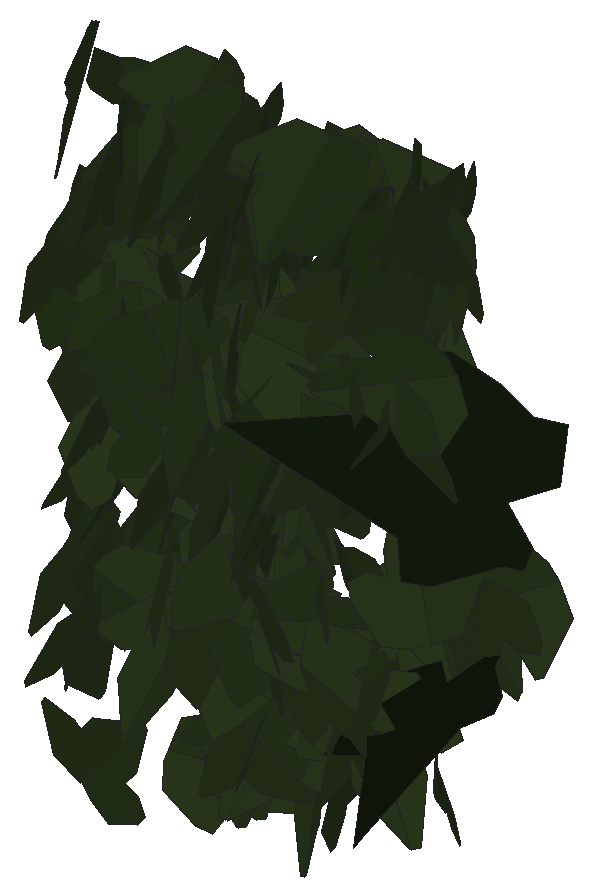
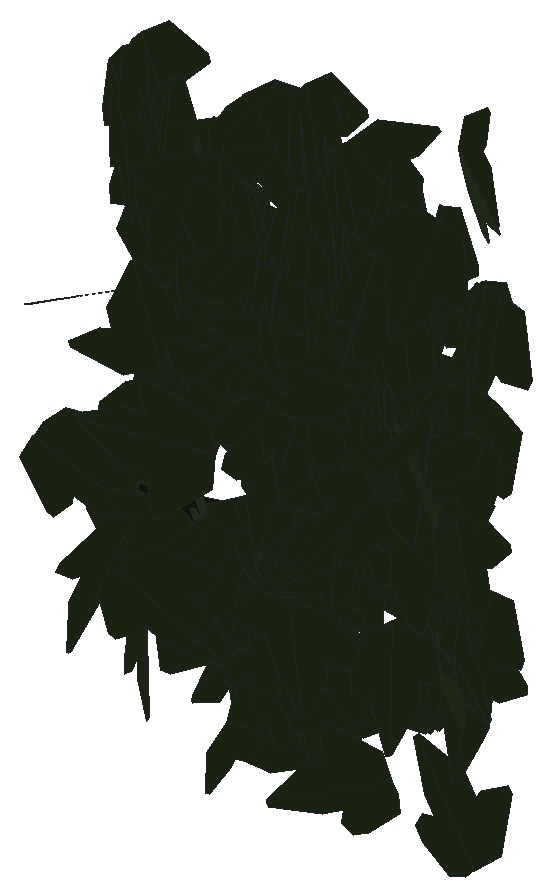
# SketchUp Ruby script. Lengths in inches.
U = 1.inch
M = Sketchup.active_model
def pt(a) = Geom::Point3d.new(a.map { |v| v * U })
def face(e, loops, mat)
  f = e.add_face(loops[0].map { |a| pt(a) })
  loops[1..].each { |l| e.add_face(l.map { |a| pt(a) }).erase! }
  f.material = f.back_material = mat if mat
  f
end
# faces: each face lists its corners as indices into pts; further lists are holes
def faces(e, pts, list, mat = nil) = list.each { |f| face(e, (f[0].is_a?(Array) ? f : [f]).map { |l| l.map { |i| pts[i] } }, mat) }
# xy, xz, yz: faces in a plane at the given z, y or x. An outline is a flat list of corners, or four numbers for a rectangle; further outlines are holes
def ring(l) = l.size == 4 ? [[l[0], l[1]], [l[2], l[1]], [l[2], l[3]], [l[0], l[3]]] : l.each_slice(2).to_a
def flat(e, list, mat, &to3) = list.each { |f| face(e, (f[0].is_a?(Array) ? f : [f]).map { |l| ring(l).map { |u, v| to3.(u, v) } }, mat) }
def xy(e, z, list, mat = nil) = flat(e, list, mat) { |x, y| [x, y, z] }
def xz(e, y, list, mat = nil) = flat(e, list, mat) { |x, z| [x, y, z] }
def yz(e, x, list, mat = nil) = flat(e, list, mat) { |y, z| [x, y, z] }
def lines(e, pts, list) = list.each { |a, b| e.add_line(pt(pts[a]), pt(pts[b])) }
# prism: a flat outline (further loops are holes) pulled along v
def prism(e, loops, v, mat = nil)
  f = face(e, loops, mat); d = Geom::Vector3d.new(v.map { |x| x * U })
  f.pushpull(f.normal.samedirection?(d) ? d.length : -d.length)
end
def box(e, o, s, mat = nil) = prism(e, [[o, [o[0] + s[0], o[1], o[2]], [o[0] + s[0], o[1] + s[1], o[2]], [o[0], o[1] + s[1], o[2]]]], [0, 0, s[2]], mat)
def at(x, y, z, deg = 0) = Geom::Transformation.translation(pt([x, y, z])) * Geom::Transformation.rotation(ORIGIN, Z_AXIS, deg.degrees)
def axes(o, x, y, z) = Geom::Transformation.new([*x, 0, *y, 0, *z, 0, *pt(o).to_a, 1])
def part(name) = M.definitions.add(name)
# library, detail: a bought-in or finely detailed component or shape, given as its bounding box
def library(name, o, s) = part(name).tap { |d| box(d.entities, o, s) }
def detail(e, o, s) = box(e.add_group.entities, o, s)
def put(e, d, t, mat = nil) = e.add_instance(d, t).tap { |i| i.material = mat if mat }
def group(e, t, mat = nil) = e.add_group.tap { |g| g.transformation = t; g.material = mat if mat }.entities
root = M.entities
M.materials.add("efeu1").color = [18, 25, 13]
M.materials.add("efeu2").color = [43, 57, 29]
c1 = part("ivyleaf_10")
p = [[0,0.5,-0.03],[-0.0625,2.02,-0.43],[-0.19,2.01,-0.46],[-0.54,1.05,-0.29],[-0.52,0.625,-0.18],[-0.83,0.76,-0.28],
  [-1.16,0.64,-0.33],[-1.15,0.33,-0.24],[-0.77,-0.39,0.02],[-0.3,-0.51,0.16],[0.04,-0.48,0.23],[-0.02,2.01,-0.4375],
  [-0.06,2.01,-0.43],[0.04,-0.49,0.23],[0.67,-0.49,0.14],[1.38,0.36,-0.2],[1.375,0.51,-0.24],[0.81,0.65,-0.19],
  [0.62,0.59,-0.15],[0.6,1.09,-0.28],[0.5,1.23,-0.31]]
faces(c1.entities,p,[[0,1,2,3,4,5,6,7,8,9,10],[11,12,0,13,14,15,16,17,18,19,20]],"efeu2")
c2 = part("ivyleaf_9")
p = [[1.54,2.16,1.25],[1.36,2.04,1.19],[-0.21,0.99,0.68],[-0.71,1.11,0.82],[-0.85,0.86,0.67],[-0.8,0.17,0.21],
  [-0.9,-0.01,0.1],[-0.67,-0.16,-0.02],[-0.08,-0.08,-0.05],[-0.03,-0.6,-0.4],[0.65,-0.88,-0.66],[0.83,-0.6,-0.49],
  [1.29,-0.42,-0.43],[1.8125,-0.07,-0.26],[1.21,0.44,0.15]]
faces(c2.entities,p,[[0,1,2,3,4,5,6,7,8,9,10,11,12,13,14]],"efeu1")
put(root,c1,axes([508.32,137.57,172.07],[0.33444,-0.46336,0.32616],[0.19775,-0.25949,-0.5714],[0.53102,0.38846,0.00736]))
put(root,c2,axes([512.88,137.89,165.84],[-0.5709,-0.44128,-0.42152],[0.64662,-0.3683,-0.39508],[0.02481,-0.55503,0.59729]))
put(root,c1,axes([513.1875,137.16,167.21],[0.1899,0.66022,-0.04458],[-0.01855,0.05168,0.68624],[0.66146,-0.18809,0.03204]))
put(root,c1,axes([511,137.58,168.73],[0.04279,-0.71118,0.27788],[0.07484,-0.27307,-0.7104],[0.75987,0.06694,0.05432]))
put(root,c2,axes([513.75,137.7,168.54],[-0.75068,0.35636,0.59387],[-0.70859,-0.54201,-0.47879],[0.16235,-0.71793,0.65625]))
put(root,c1,axes([510.41,136.8,166.26],[0.02054,-0.16896,-0.72847],[0.26646,0.68257,-0.15081],[0.69873,-0.25533,0.07892]))
put(root,c1,axes([511.78,137.48,169.28],[0.48375,-0.23299,0.34543],[0.34148,-0.08161,-0.53325],[0.23875,0.5888,0.06278]))
put(root,c1,axes([510.8,136.99,169.16],[-0.21497,0.24459,0.55114],[-0.42952,0.35297,-0.32478],[-0.46136,-0.44257,0.04557]))
put(root,c1,axes([511.97,137.625,165.58],[0.2065,-0.37848,-0.50768],[0.33346,-0.38896,0.42561],[-0.53832,-0.38612,0.06889]))
put(root,c1,axes([510.77,137.26,166.55],[-0.60109,0.4031,-0.03478],[0.02781,-0.02096,-0.72373],[-0.40364,-0.60173,0.00192]))
put(root,c1,axes([511.95,137.25,168.6],[-0.24629,-0.56282,-0.21689],[0.09421,0.19551,-0.61431],[0.59577,-0.26359,0.00747]))
put(root,c1,axes([509.11,137.61,167.84],[-0.25404,0.46707,0.36591],[0.11994,-0.3494,0.52927],[0.58109,0.27632,0.05073]))
put(root,c1,axes([510.3,137.42,170.68],[0.23232,-0.59093,-0.06122],[0.01744,0.07249,-0.63353],[0.59384,0.22905,0.04256]))
put(root,c1,axes([510.21,137.71,167.7],[0.13338,-0.60424,0.29815],[0.09615,-0.28376,-0.61808],[0.6669,0.16176,0.02948]))
put(root,c1,axes([511.46,137.47,165.78],[-0.28082,0.01322,-0.60596],[0.58482,-0.16953,-0.27472],[-0.15922,-0.646,0.05969]))
put(root,c1,axes([511,137.19,166.1875],[-0.31425,-0.21352,-0.5687],[0.51862,0.23908,-0.37634],[0.31629,-0.60416,0.05206]))
put(root,c1,axes([513.11,137.35,168.99],[-0.23811,0.01834,0.63],[-0.63026,-0.00386,-0.2381],[-0.00288,-0.67348,0.01852]))
put(root,c1,axes([512.95,137.49,169.77],[0.25306,0.09367,-0.64986],[-0.65654,0.04326,-0.24943],[0.00675,0.69605,0.10296]))
put(root,c1,axes([508.4,137.82,165.85],[0.24396,-0.4976,0.40781],[0.20164,-0.35503,-0.55383],[0.61095,0.31588,0.01995]))
put(root,c1,axes([510.9,137.26,164.86],[-0.34113,-0.40429,-0.35378],[0.24067,0.25966,-0.5288],[0.4803,-0.41725,0.01371]))
put(root,c1,axes([508.52,137.38,165.39],[-0.08968,-0.61593,-0.20414],[0.03086,0.2018,-0.62243],[0.64815,-0.09483,0.00139]))
put(root,c1,axes([509.37,137.84,165.36],[-0.23349,-0.48068,0.35286],[0.02561,-0.38668,-0.50981],[0.59574,-0.17177,0.16021]))
put(root,c1,axes([510.66,137.26,165.49],[0.27765,0.31305,0.44729],[0.24955,0.36454,-0.4196],[-0.51748,0.34376,0.03765]))
put(root,c1,axes([511.26,137.82,171.72],[-0.36212,-0.44252,0.31408],[-0.08731,-0.32515,-0.5588],[0.53558,-0.35221,0.12126]))
put(root,c1,axes([510.59,137.6,171.95],[0.06581,-0.66166,-0.0581],[0.00212,0.0586,-0.66488],[0.66421,0.06537,0.00788]))
put(root,c1,axes([508.23,137.41,170.1],[0.13259,-0.58806,-0.3005],[0.04504,0.31383,-0.59429],[0.65885,0.09689,0.1011]))
put(root,c1,axes([510.93,137.69,167.89],[0.3619,-0.12328,0.46846],[0.49098,-0.04076,-0.36333],[0.11542,0.55993,0.07669]))
put(root,c1,axes([512.94,137.65,171.84],[-0.00539,-0.64528,-0.01357],[0.00112,0.01356,-0.6453],[0.64542,-0.00541,0.00101]))
put(root,c1,axes([508.81,137.54,165.85],[-0.35451,-0.05588,-0.47064],[0.48814,0.03373,-0.34529],[0.065,-0.55803,0.02626]))
put(root,c1,axes([508.31,137.69,163.3],[-0.50719,-0.02251,0.41112],[0.40969,0.03734,0.50747],[-0.04098,0.65182,-0.01487]))
put(root,c1,axes([508.3,137.41,166.08],[-0.04211,-0.52875,-0.38857],[0.12038,0.37654,-0.52541],[0.64503,-0.10479,0.07269]))
put(root,c1,axes([511.05,137.87,171.66],[-0.26447,-0.53912,0.25266],[-0.05782,-0.2519,-0.59802],[0.59257,-0.26519,0.05441]))
put(root,c1,axes([513.29,137.64,171.3125],[0.47803,-0.41019,-0.22241],[-0.16696,0.14696,-0.62989],[0.43571,0.50634,0.00265]))
put(root,c1,axes([512.46,137.38,168.9375],[-0.00828,-0.5128,-0.43211],[0.03155,0.43136,-0.51252],[0.66984,-0.02666,0.0188]))
put(root,c1,axes([508.26,137.32,169.92],[-0.09979,-0.48567,-0.50798],[0.11047,0.49585,-0.49578],[0.69406,-0.14875,0.00587]))
put(root,c1,axes([510.72,137.57,164.9375],[0.23264,-0.49703,-0.25784],[-0.09762,0.23101,-0.56331],[0.59188,0.23346,0.00844]))
put(root,c1,axes([511.24,137.29,166.3],[0.09838,0.03395,0.63404],[0.30837,0.55831,-0.07774],[-0.55504,0.3162,0.06919]))
put(root,c1,axes([512.77,137.68,170.73],[-0.23079,-0.59385,-0.05254],[0.01187,0.05175,-0.63708],[0.59606,-0.23097,-0.00765]))
put(root,c1,axes([509.87,137.86,168.3],[-0.22774,-0.52677,0.20534],[-0.07468,-0.18499,-0.59009],[0.60295,-0.22187,0.00447]))
put(root,c1,axes([513.31,137.52,171.5],[-0.46821,0.21017,0.39693],[-0.38489,0.10775,-0.51106],[-0.23148,-0.60428,0.04692]))
put(root,c1,axes([509.23,137.61,169.03],[-0.46464,-0.40945,-0.19416],[0.17101,0.10402,-0.61677],[0.45492,-0.4573,0.03355]))
put(root,c1,axes([509.17,137.71,166.17],[0.47328,-0.42678,-0.18837],[-0.12982,0.13725,-0.63712],[0.44808,0.49055,0.01438]))
put(root,c1,axes([509.5,138.04,171.89],[-0.21548,-0.49068,0.35974],[-0.00841,-0.3792,-0.52226],[0.60837,-0.17904,0.1202]))
put(root,c1,axes([508.29,137.75,167.17],[0.06494,-0.57052,-0.05626],[-0.00521,0.05389,-0.59662],[0.6189,0.06032,0.00088]))
put(root,c1,axes([508.67,137.59,168.07],[0.06405,-0.60995,-0.29481],[-0.04619,0.2915,-0.61315],[0.67588,0.07772,-0.01397]))
put(root,c1,axes([511.01,137.95,167.11],[-0.26619,0.32371,-0.48857],[0.27976,-0.40133,-0.41833],[-0.51499,-0.38534,0.02527]))
put(root,c1,axes([511.95,137.88,165.3],[-0.6803,-0.21481,-0.27284],[0.35624,-0.26001,-0.60226],[0.08482,-0.63088,0.34111]))
put(root,c1,axes([508.6875,137.58,170.98],[0.19561,-0.59786,-0.34202],[-0.02589,0.34891,-0.62472],[0.68829,0.18304,0.0737]))
put(root,c1,axes([510.7,137.83,164.75],[0.61692,0.0313,-0.20388],[-0.2036,-0.01063,-0.61771],[-0.03306,0.64965,-0.00028]))
put(root,c1,axes([511.13,137.36,169.58],[0.15039,0.31893,0.58519],[0.229,0.53865,-0.35242],[-0.62588,0.27372,0.01167]))
put(root,c1,axes([511.77,138.02,168.46],[-0.40263,-0.17656,-0.50346],[-0.45688,-0.21161,0.43959],[-0.27551,0.60894,0.00679]))
put(root,c1,axes([509.78,138.16,171.51],[-0.02859,-0.46082,0.44097],[0.01007,-0.44168,-0.46091],[0.63773,-0.01368,0.02705]))
put(root,c1,axes([510.59,137.7,171.64],[0.25359,-0.56911,-0.22876],[-0.05494,0.22547,-0.62183],[0.6109,0.25652,0.03903]))
put(root,c1,axes([508.67,137.5625,167.65],[0.31685,0.32075,0.47654],[0.34424,0.32965,-0.45077],[-0.45986,0.46778,-0.00909]))
put(root,c1,axes([509.43,137.51,171.26],[0.09444,-0.52721,-0.47273],[-0.00729,0.47617,-0.5325],[0.70808,0.07522,0.05757]))
put(root,c1,axes([511.07,137.98,164.36],[0.49749,-0.29093,0.2424],[0.21312,-0.12404,-0.56661],[0.34157,0.50113,0.00048]))
put(root,c1,axes([509.62,137.91,168.69],[-0.4539,0.29887,-0.29941],[0.18596,-0.24722,-0.52832],[-0.40777,-0.44542,0.09234]))
put(root,c1,axes([510.25,137.875,165.66],[-0.08161,-0.05283,0.62763],[0.65376,0.01717,0.08039],[-0.02556,0.60796,0.05227]))
put(root,c1,axes([511.55,138.15,168.125],[-0.29378,-0.41075,0.42034],[-0.10875,-0.42382,-0.49016],[0.57756,-0.28873,0.12152]))
put(root,c1,axes([510.82,137.82,167.625],[0.2129,-0.64095,-0.14218],[-0.05377,0.13194,-0.67532],[0.65432,0.21939,-0.00924]))
put(root,c1,axes([510.31,137.93,164.72],[-0.19437,-0.54076,0.05967],[0.07114,-0.08167,-0.58563],[0.58297,-0.17033,0.09136]))
put(root,c1,axes([510.91,137.75,168.83],[0.57655,0.28141,0.05878],[-0.05944,-0.0122,0.64139],[0.28128,-0.57941,0.01505]))
put(root,c1,axes([511.86,137.38,164.57],[-0.0036,-0.08927,-0.63569],[-0.03046,0.635,-0.089],[0.6412,0.02967,-0.0078]))
put(root,c1,axes([511.62,138.05,171.04],[-0.08297,-0.61818,0.16046],[0.05561,-0.16819,-0.61919],[0.63624,-0.06592,0.07505]))
put(root,c1,axes([509.875,137.91,168],[0.03745,0.04221,-0.58788],[-0.61196,0.01799,-0.03475],[0.01666,0.56605,0.04495]))
put(root,c1,axes([511.63,138.05,170.19],[-0.18536,-0.61522,0.17697],[-0.0332,-0.17475,-0.64229],[0.63931,-0.18745,0.01796]))
put(root,c1,axes([510.25,137.96,164.41],[-0.37928,-0.4383,0.0717],[0.0323,-0.11111,-0.57619],[0.47809,-0.34021,0.09581]))
put(root,c1,axes([508.41,137.51,168.57],[-0.14682,-0.2353,-0.60205],[0.30525,0.51896,-0.27727],[0.56977,-0.33866,-0.00659]))
put(root,c1,axes([508.51,138.33,167.31],[0.0904,-0.53137,0.45675],[0.07177,-0.45109,-0.53899],[0.69701,0.11537,-0.00374]))
put(root,c1,axes([511.74,138.07,171.14],[0.22497,-0.60375,0.02625],[0.00988,-0.02433,-0.6443],[0.60424,0.22519,0.00076]))
put(root,c1,axes([509.33,137.82,169.23],[0.41224,-0.44987,-0.32144],[-0.08529,0.34442,-0.5914],[0.54629,0.39325,0.15023]))
put(root,c1,axes([508.52,137.78,166],[0.26467,-0.15479,-0.55967],[-0.42326,0.36966,-0.3024],[0.39755,0.49662,0.05065]))
put(root,c1,axes([508.69,137.7,168.5],[0.16145,-0.43353,-0.48199],[-0.05489,0.48579,-0.45534],[0.64595,0.14964,0.08178]))
put(root,c1,axes([512.09,138.02,171.1],[-0.24763,-0.6144,-0.03144],[0.011,0.02946,-0.66242],[0.6151,-0.24787,-0.00081]))
put(root,c1,axes([509.35,137.7,167.4],[-0.01958,-0.46523,-0.47929],[0.04362,0.47758,-0.46535],[0.66652,-0.04492,0.01637]))
put(root,c1,axes([509.92,138.08,170.77],[0.04985,-0.63913,-0.08309],[0.00924,0.08404,-0.64088],[0.64444,0.04823,0.01562]))
put(root,c1,axes([508.08,138.03,168.63],[-0.41685,-0.02818,-0.48224],[0.50023,0.02302,-0.40242],[0.03859,-0.60288,0.00718]))
put(root,c1,axes([510.55,137.97,170.74],[0.02848,-0.5821,-0.28606],[0.0531,0.28747,-0.57968],[0.64642,0.00203,0.06022]))
put(root,c1,axes([510.37,137.81,170.52],[-0.24274,0.35034,0.46438],[-0.36075,0.30662,-0.42506],[-0.49556,-0.39482,0.08196]))
put(root,c1,axes([507.96,137.97,168.99],[-0.36707,-0.23463,-0.47744],[0.44992,0.17258,-0.43072],[0.28385,-0.57698,0.06531]))
put(root,c1,axes([510.32,138.52,169.82],[0.07768,-0.49211,0.4212],[0.11833,-0.4063,-0.49652],[0.63685,0.13552,0.04088]))
put(root,c1,axes([512.32,138.02,171.6],[0.20122,-0.5402,-0.28923],[0.00328,0.30537,-0.56806],[0.61274,0.17576,0.09803]))
put(root,c1,axes([510.66,138.25,168.31],[0.47875,0.34345,-0.1365],[-0.11766,-0.07366,-0.58314],[-0.37926,0.4564,0.00861]))
put(root,c1,axes([509.51,137.98,163.76],[0.14572,0.10615,0.56483],[0.45905,0.33808,-0.17854],[-0.3827,0.44595,0.00091]))
put(root,c1,axes([512.84,138.19,171.5],[0.15055,-0.62247,-0.10999],[0.02835,0.1196,-0.63806],[0.63148,0.14303,0.05487]))
put(root,c1,axes([513.2,138.18,166.9375],[-0.60563,-0.08738,0.19608],[-0.19051,-0.05166,-0.61147],[0.09891,-0.63448,0.02279]))
put(root,c1,axes([512.86,137.92,164.82],[-0.29478,0.23975,0.51389],[-0.44156,0.26634,-0.37754],[-0.35579,-0.52919,0.0428]))
put(root,c1,axes([510.46,138.2,168.83],[-0.61927,-0.07095,-0.04556],[0.05513,-0.05798,-0.59723],[0.07121,-0.57214,0.06617]))
put(root,c1,axes([509.28,138.41,167.25],[-0.05874,0.47684,-0.31886],[-0.17114,-0.30851,-0.46978],[-0.58785,0.04217,0.16863]))
put(root,c1,axes([509.5,138.1875,167.66],[0.44465,0.40997,0.06782],[0.05094,0.04505,-0.60426],[-0.44543,0.41441,-0.00141]))
put(root,c1,axes([510.88,138.42,170.86],[-0.35449,0.26322,-0.40531],[0.21685,-0.35132,-0.42265],[-0.45929,-0.36904,0.11327]))
put(root,c1,axes([509.03,137.93,170.8],[-0.19111,-0.41764,-0.47317],[0.22821,0.4152,-0.45864],[0.58841,-0.29667,0.0242]))
put(root,c1,axes([510.3,137.75,167.17],[0.11566,-0.09608,-0.65701],[-0.0171,0.66625,-0.10044],[0.66377,0.03391,0.11189]))
put(root,c1,axes([510.76,138.25,168.21],[0.57089,0.20392,-0.10079],[-0.1345,0.05754,-0.58052],[-0.20339,0.53432,0.10099]))
put(root,c1,axes([510.09,137.88,164.18],[0.04748,-0.04763,-0.65548],[0.48598,0.44496,0.00287],[0.44243,-0.48365,0.06719]))
put(root,c1,axes([510.14,138.08,168.77],[0.28482,0.4654,0.27429],[0.1488,0.22503,-0.55626],[-0.55824,0.29744,-0.00832]))
put(root,c1,axes([510.64,137.98,170.65],[0.19077,-0.38358,-0.48797],[-0.08196,0.49046,-0.41758],[0.61524,0.18427,0.09567]))
put(root,c1,axes([509.79,138.26,171.73],[0.466,-0.43154,-0.11851],[0.00627,0.17737,-0.62123],[0.44747,0.44692,0.13212]))
put(root,c1,axes([509.9,138.18,170.82],[-0.0905,-0.59805,-0.24266],[0.02603,0.24145,-0.60478],[0.64488,-0.09367,-0.00964]))
put(root,c1,axes([508.29,137.93,168.91],[-0.0413,-0.18001,-0.6576],[0.44851,0.48901,-0.16203],[0.5135,-0.4416,0.08863]))
put(root,c1,axes([509.33,138.23,170.62],[-0.39556,0.50227,0.0222],[-0.01202,0.01879,-0.63932],[-0.50262,-0.39573,-0.00218]))
put(root,c1,axes([511.16,138.71,171.22],[-0.1384,-0.36078,0.41899],[-0.00046,-0.41396,-0.38568],[0.58407,-0.08582,0.09898]))
put(root,c1,axes([508.74,138.37,170.8],[-0.3804,-0.51311,-0.08072],[0.07659,0.04355,-0.63776],[0.51374,-0.38643,0.03531]))
put(root,c1,axes([508.625,138.42,170.43],[-0.26477,-0.57937,-0.00286],[-0.00275,0.0044,-0.63699],[0.57937,-0.26475,-0.00433]))
put(root,c1,axes([509.49,138.5,166.85],[0.50747,0.26058,-0.16219],[-0.13664,-0.09322,-0.55843],[-0.29816,0.48623,-0.02014]))
put(root,c1,axes([510.45,138.4,167.84],[-0.60255,0.04015,-0.0519],[0.05182,-0.02789,-0.58119],[-0.04582,-0.55945,0.02525]))
put(root,c1,axes([512.35,138.29,168.57],[0.55119,0.35634,-0.13418],[0.10775,0.08045,0.65628],[0.3652,-0.56155,0.00888]))
put(root,c1,axes([508.32,138.4,171.375],[-0.62666,0.07208,-0.12786],[0.12816,-0.00456,-0.63072],[-0.07154,-0.63956,-0.00991]))
put(root,c1,axes([508.34,138.46,167.97],[0.22185,-0.52852,0.09028],[-0.0305,0.08215,0.58971],[-0.57765,-0.20732,0.00353]))
put(root,c1,axes([513.5,138.57,166.96],[0.35047,0.02989,-0.56874],[-0.56952,0.01961,-0.34992],[0.00104,0.66776,0.03573]))
put(root,c1,axes([511.01,138.67,171.27],[-0.54949,0.19117,-0.12321],[0.04476,-0.20832,-0.5347],[-0.23874,-0.47906,0.18334]))
put(root,c1,axes([509.03,138.27,167.93],[-0.24492,-0.38922,-0.54398],[0.35115,0.41823,-0.45734],[0.5693,-0.42542,0.04807]))
put(root,c1,axes([509.71,138.36,169.15],[-0.14002,-0.16451,0.54078],[0.35771,0.40087,0.21779],[-0.46795,0.35566,0.00467]))
put(root,c1,axes([510.79,138.65,170.55],[-0.47161,0.05587,-0.35812],[0.34798,-0.14687,-0.44972],[-0.14441,-0.53636,0.08584]))
put(root,c1,axes([511.85,138.5,166.41],[0.42472,0.20292,0.45096],[0.39046,0.22718,-0.46996],[-0.30345,0.57632,0.02647]))
put(root,c1,axes([509.3,138.62,165.64],[0.24688,-0.06603,-0.52395],[-0.53221,0.10582,-0.24697],[0.13374,0.54302,-0.01558]))
put(root,c1,axes([511.2,138.61,166.33],[-0.54907,0.31547,-0.19176],[0.16135,-0.10406,-0.63318],[-0.33206,-0.57221,0.00942]))
put(root,c1,axes([508.25,138.22,169.25],[0.19941,-0.21733,-0.57255],[0.17638,0.597,-0.16518],[0.58646,-0.10566,0.24436]))
put(root,c1,axes([511.3125,138.53,171.08],[0.45512,0.34796,0.36773],[0.28676,0.23032,-0.57285],[-0.41722,0.53787,0.00741]))
put(root,c1,axes([510.55,139.07,164.68],[0.0814,0.36895,-0.52964],[-0.08922,-0.52228,-0.37753],[-0.63928,0.11987,-0.01475]))
put(root,c1,axes([508.52,138.75,166.16],[-0.17669,-0.51915,-0.11302],[0.01384,0.10982,-0.5657],[0.57267,-0.16283,-0.0212]))
put(root,c1,axes([512,138.98,165.92],[0.48437,0.07712,-0.4767],[-0.4693,-0.08395,-0.49043],[-0.11381,0.6744,-0.00653]))
put(root,c1,axes([510.03,139.07,165.23],[0.19379,-0.02855,0.63402],[0.61568,-0.15246,-0.19505],[0.15406,0.64521,-0.01804]))
put(root,c1,axes([511.47,138.87,167.84],[-0.02645,0.01832,-0.68042],[0.67959,-0.0376,-0.02743],[-0.0383,-0.6799,-0.01681]))
put(root,c1,axes([509.66,139.09,166.29],[0.64947,0.10897,0.06347],[0.06229,0.0123,-0.65854],[-0.10965,0.65244,0.00181]))
put(root,c1,axes([512.42,138.93,166.31],[-0.07238,0.63015,0.26909],[-0.02304,0.26819,-0.63425],[-0.68481,-0.07562,-0.0071]))
